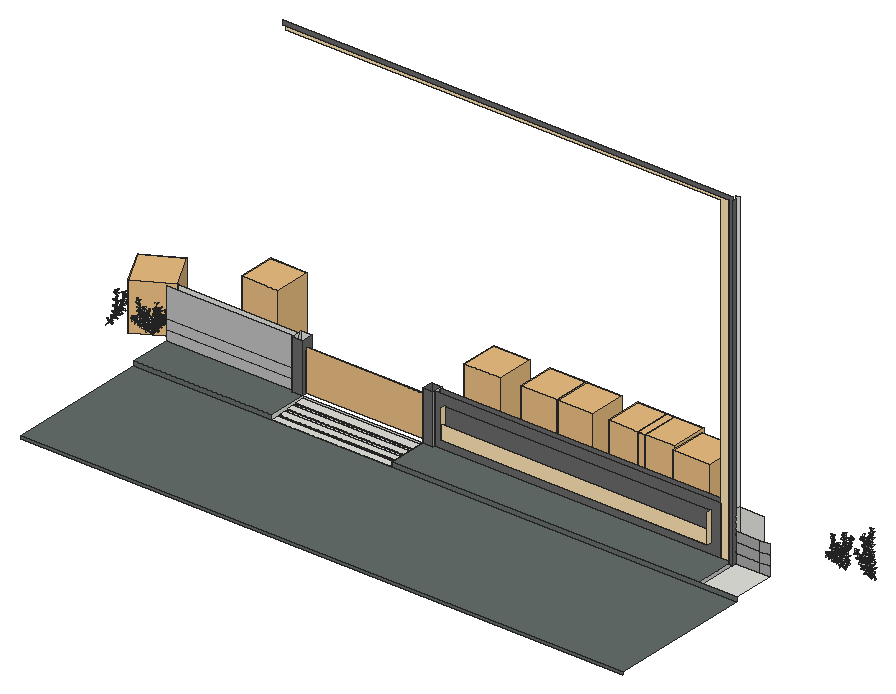
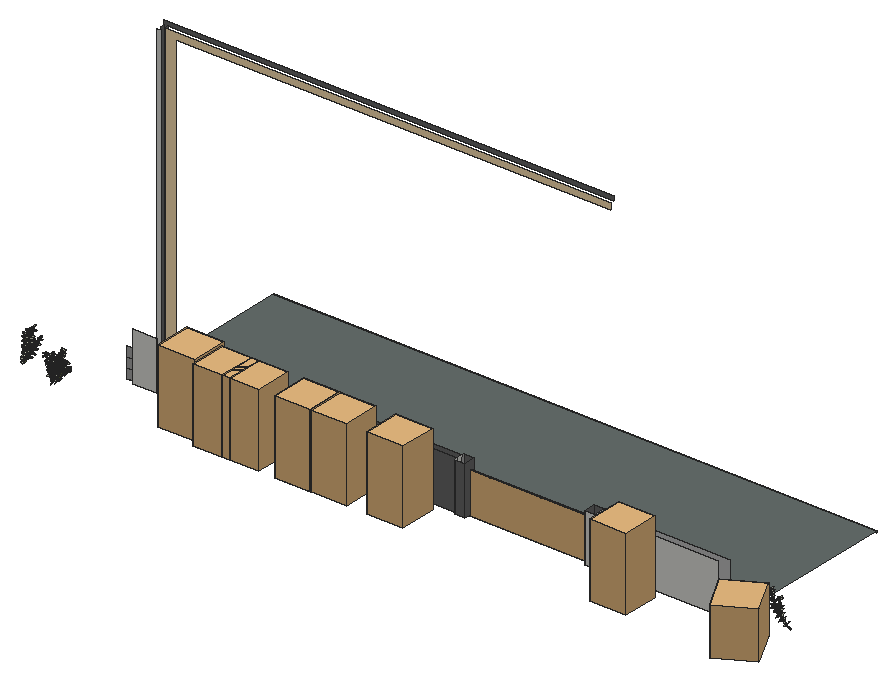
# SketchUp Ruby script. Lengths in inches.
U = 1.inch
M = Sketchup.active_model
def pt(a) = Geom::Point3d.new(a.map { |v| v * U })
def face(e, loops, mat)
  f = e.add_face(loops[0].map { |a| pt(a) })
  loops[1..].each { |l| e.add_face(l.map { |a| pt(a) }).erase! }
  f.material = f.back_material = mat if mat
  f
end
# faces: each face lists its corners as indices into pts; further lists are holes
def faces(e, pts, list, mat = nil) = list.each { |f| face(e, (f[0].is_a?(Array) ? f : [f]).map { |l| l.map { |i| pts[i] } }, mat) }
# xy, xz, yz: faces in a plane at the given z, y or x. An outline is a flat list of corners, or four numbers for a rectangle; further outlines are holes
def ring(l) = l.size == 4 ? [[l[0], l[1]], [l[2], l[1]], [l[2], l[3]], [l[0], l[3]]] : l.each_slice(2).to_a
def flat(e, list, mat, &to3) = list.each { |f| face(e, (f[0].is_a?(Array) ? f : [f]).map { |l| ring(l).map { |u, v| to3.(u, v) } }, mat) }
def xy(e, z, list, mat = nil) = flat(e, list, mat) { |x, y| [x, y, z] }
def xz(e, y, list, mat = nil) = flat(e, list, mat) { |x, z| [x, y, z] }
def yz(e, x, list, mat = nil) = flat(e, list, mat) { |y, z| [x, y, z] }
def lines(e, pts, list) = list.each { |a, b| e.add_line(pt(pts[a]), pt(pts[b])) }
# prism: a flat outline (further loops are holes) pulled along v
def prism(e, loops, v, mat = nil)
  f = face(e, loops, mat); d = Geom::Vector3d.new(v.map { |x| x * U })
  f.pushpull(f.normal.samedirection?(d) ? d.length : -d.length)
end
def box(e, o, s, mat = nil) = prism(e, [[o, [o[0] + s[0], o[1], o[2]], [o[0] + s[0], o[1] + s[1], o[2]], [o[0], o[1] + s[1], o[2]]]], [0, 0, s[2]], mat)
def at(x, y, z, deg = 0) = Geom::Transformation.translation(pt([x, y, z])) * Geom::Transformation.rotation(ORIGIN, Z_AXIS, deg.degrees)
def axes(o, x, y, z) = Geom::Transformation.new([*x, 0, *y, 0, *z, 0, *pt(o).to_a, 1])
def part(name) = M.definitions.add(name)
# library, detail: a bought-in or finely detailed component or shape, given as its bounding box
def library(name, o, s) = part(name).tap { |d| box(d.entities, o, s) }
def detail(e, o, s) = box(e.add_group.entities, o, s)
def put(e, d, t, mat = nil) = e.add_instance(d, t).tap { |i| i.material = mat if mat }
def group(e, t, mat = nil) = e.add_group.tap { |g| g.transformation = t; g.material = mat if mat }.entities
root = M.entities
M.materials.add("0ad16as01f6asdLeafVar1sfd015as60f1as6").color = [231, 235, 211]
M.materials.add("[0032_Moccasin]").color = [255, 228, 181]
M.materials.add("[0131_Silver]").color = [192, 192, 192]
M.materials.add("[0132_LightGray]").color = [169, 169, 169]
M.materials.add("[0134_DimGray]").color = [105, 105, 105]
M.materials.add("[Marble Carrara Gold Floor Tile]").color = [225, 223, 217]
M.materials.add("[Slate]").color = [102, 110, 108]
M.materials.add("asdfasdf0165f6asdLeafVar1sfd015as60f1as6").color = [231, 235, 211]
M.materials.add("dw_stemssadfasdfa0sdf1s01d6w1").color = [90, 97, 50]
c1 = part("vdw_leaf\#2")
p = [[0,0,0],[-2.77,1.61,2.32],[-4.3125,6.1,4.5],[-3.97,13.49,6.09],[-2.47,18.57,6.3],[-0.2,22.73,5.75],
  [2.54,19.66,6.85],[4.3,15.93,7.09],[5.03,7.6,5.43],[3.32,1.76,2.74]]
faces(c1.entities,p,[[0,1,2,3,4,5],[0,5,6,7,8,9]],"asdfasdf0165f6asdLeafVar1sfd015as60f1as6")
c2 = part("dg_branch_1\#2")
p = [[46.12,1.57,35.62],[46,5.42,35.41],[0.14,1.79,0.05],[0.26,-2.0625,0.27],[74.05,2.99,75.8],[74.11,5.28,75.58],
  [103.46,0.47,94.74],[104.03,2.92,94.84],[81.14,16.92,120.46],[81.2,18.78,120.24],[130.47,-5.6875,130.27],[130.58,-3.66,129.85],
  [80.82,34.4375,191.22],[80.64,35.93,190.9],[148.49,-14.56,203.24],[148.9,-12.8125,203.11],[81.08,37.95,226.93],[81.4,39.1,227.03],
  [157.45,-18.19,250.77],[157.7,-17.01,250.41]]
faces(c2.entities,p,[[0,1,2,3],[4,0,1],[4,1,5],[6,4,5],[6,5,7],[8,4,5],[8,5,9],[10,6,7],
  [10,7,11],[12,8,9],[12,9,13],[14,10,11],[14,11,15],[16,12,13],[16,13,17],[18,14,15],
  [18,15,19]],"dw_stemssadfasdfa0sdf1s01d6w1")
c3 = part("vdw_branch1\#3")
put(c3.entities,c1,axes([120.69,-2.42,117.31],[1.12221,-0.24063,-0.65809],[0.19207,1.24776,-0.12871],[0.65778,0.01392,1.11658]))
put(c3.entities,c1,axes([81,38.9,226.05],[0.7888,-0.58155,0],[0.48308,0.65523,0.47],[-0.28484,-0.38635,0.83138]))
put(c3.entities,c1,axes([78.08,12.69,106.05],[-1.43826,-0.02353,-0.03177],[0.0088,-1.31777,0.57755],[-0.03854,0.57714,1.31741]))
put(c3.entities,c1,axes([130.18,-4.73,130.41],[-0.38031,-1.29044,-0.11242],[1.20662,-0.31032,-0.51987],[0.47109,-0.24694,1.24081]))
put(c3.entities,c1,axes([157.08,-17.89,249.93],[-0.91355,0.40674,0],[-0.37496,-0.84216,0.38752],[0.15762,0.35401,0.92186]))
put(c3.entities,c1,axes([90.64,3.03,86.49],[0.32514,-0.85045,-0.99675],[0.69523,0.98247,-0.61148],[1.11061,-0.36604,0.67459]))
put(c3.entities,c1,axes([80.15,28.42,160.95],[-0.16039,0.95636,-1.06292],[-1.41646,0.03966,0.24943],[0.19509,1.07422,0.93709]))
put(c3.entities,c1,axes([126.74,-5.45,129.22],[-0.59819,0.96152,-0.6841],[-0.85772,0.12575,0.92675],[0.75427,0.88089,0.57856]))
put(c3.entities,c1,axes([133.22,-6.12,150.66],[-0.93823,0.76985,0.59124],[-0.47726,-1.08188,0.65135],[0.84525,0.24366,1.02405]))
put(c3.entities,c1,axes([80.43,22.89,141.32],[-1.42571,-0.19312,0.01373],[0.18338,-1.31425,0.5561],[-0.0621,0.5528,1.32692]))
put(c3.entities,c1,axes([33.14,0.88,26.42],[-0.13338,1.31536,0.04876],[-1.04528,-0.13221,0.7073],[0.72315,0.03348,1.07497]))
put(c3.entities,c1,axes([152.63,-15.08,221.76],[-1.28188,0.41945,0.0579],[-0.3638,-1.18547,0.53367],[0.21665,0.49113,1.23869]))
put(c3.entities,c1,axes([80.05,28.28,160.33],[-0.46732,-1.26661,0.40679],[1.27397,-0.40257,0.21004],[-0.07408,0.44645,1.30501]))
put(c3.entities,c1,axes([153.95,-14.8,235.875],[0.39005,1.07743,0.20605],[-0.96443,0.25296,0.50293],[0.42961,-0.3464,0.99807]))
put(c3.entities,c1,axes([80.2,24.22,141.74],[1.33062,-0.46576,0.02628],[0.44746,1.2746,-0.06608],[-0.00197,0.0722,1.37936]))
put(c3.entities,c1,axes([145.48,-12.5,188.92],[-1.32952,0.16983,0.16138],[-0.09299,-1.2361,0.53471],[0.21503,0.51548,1.22904]))
put(c3.entities,c1,axes([139.64,-9.18,171.24],[0.05682,1.30088,0.23414],[-1.13176,-0.05343,0.57151],[0.58357,-0.22963,1.13417]))
put(c3.entities,c1,axes([70.95,4.35,71.98],[-1.1081,-0.41873,0.64752],[0.33675,-1.28259,-0.25313],[0.6937,-0.04625,1.15721]))
put(c3.entities,c1,axes([59.85,4.55,56.17],[-0.26797,1.24526,0.35754],[-0.9369,-0.41634,0.74783],[0.83377,-0.10389,0.98674]))
put(c3.entities,c1,axes([33.11,3.36,25.66],[-0.57817,-1.07968,-0.5679],[1.11554,-0.21356,-0.7297],[0.49375,-0.78178,0.98363]))
put(c3.entities,c2,at(-0.21,0.34,-0.17),"dw_stemssadfasdfa0sdf1s01d6w1")
put(c3.entities,c1,axes([80.91,19.01,122.53],[-0.84258,1.13222,-0.27981],[-1.15093,-0.75138,0.42537],[0.18861,0.47293,1.3457]))
put(c3.entities,c1,axes([119.8,-1.22,114.1],[-1.3235,-0.25012,0.09101],[0.25933,-1.31572,0.15537],[0.05991,0.1698,1.33794]))
put(c3.entities,c1,axes([46.29,5.1,38.04],[0.98937,0.73827,-0.47585],[-0.72359,1.03721,0.10473],[0.44068,0.18581,1.20453]))
put(c3.entities,c1,axes([81.1875,33.03,184.45],[1.33883,0.26986,0.35053],[-0.09581,1.22087,-0.57399],[-0.42216,0.53228,1.20262]))
put(c3.entities,c1,axes([80.16,36.28,206.98],[-0.83993,0.85737,-0.6234],[-1.05964,-0.65701,0.5241],[0.02941,0.81391,1.07976]))
put(c3.entities,c1,axes([154.86,-16.15,234.87],[0.02509,-1.15302,-0.28506],[1.1487,-0.04894,0.29908],[-0.30202,-0.28195,1.11384]))
put(c3.entities,c1,axes([108.77,-0.33,101.14],[-0.47691,-1.03266,-0.72709],[1.25395,-0.29455,-0.40416],[0.15052,-0.81814,1.06325]))
put(c3.entities,c1,axes([89.79,3.01,85.87],[-0.61344,0.75518,0.8965],[-0.17758,-1.01824,0.73622],[1.13385,0.22574,0.58569]))
put(c3.entities,c1,axes([81.56,20.31,123.29],[0.37259,-1.3435,0.21057],[1.29385,0.32364,-0.22445],[0.16906,0.25791,1.34638]))
put(c3.entities,c1,axes([46.45,1.82,36.74],[-0.77883,0.29892,1.0614],[0.19124,-1.24314,0.49044],[1.08598,0.43329,0.67484]))
put(c3.entities,c1,axes([71.37,4.02,72.32],[0.72905,0.81546,-0.74421],[-0.66805,0.98958,0.42988],[0.8391,0.14186,0.97745]))
put(c3.entities,c1,axes([136.59,-5.88,150.53],[0.85845,-0.99897,-0.12437],[0.96526,0.81273,0.13453],[-0.02572,-0.18182,1.28292]))
put(c3.entities,c1,axes([80.375,38.8,225.86],[-0.25178,0.96778,0],[-0.89216,-0.23211,0.38752],[0.37503,0.09757,0.92186]))
put(c3.entities,c1,axes([74.43,7.99,85.38],[-1.05703,0.91669,-0.33543],[-0.95806,-0.87958,0.61531],[0.18697,0.6754,1.25659]))
put(c3.entities,c1,axes([76.57,9.74,89.32],[0.63146,-1.21538,0.33508],[1.18148,0.49387,-0.43517],[0.26321,0.48577,1.26593]))
put(c3.entities,c1,axes([81.6875,36.97,207.4],[0.09422,-1.04424,0.38486],[1.01646,0.1939,0.27727],[-0.33299,0.33382,0.98727]))
put(c3.entities,c1,axes([157.29,-17.17,249.98],[0.50586,-0.50586,0],[0.38853,0.38853,0.41105],[-0.29684,-0.29684,0.56115]))
put(c3.entities,c1,axes([79.92,15.8,106.09],[1.03917,-0.29343,-0.90675],[-0.14587,1.22131,-0.5624],[0.92163,0.5191,0.88824]))
put(c3.entities,c1,axes([61.95,3.88,56.26],[0.41243,-1.28546,0],[1.17466,0.37688,-0.54831],[0.5221,0.16751,1.23363]))
put(c3.entities,c1,axes([151.99,-14.79,208.15],[-0.48571,-1.21723,-0.32393],[1.25386,-0.50033,0],[-0.12005,-0.30087,1.31056]))
put(c3.entities,c1,axes([108.44,0.62,102.22],[0.82183,0.96078,0.38967],[-0.62327,0.08618,1.10203],[0.79141,-0.88661,0.51693]))
put(c3.entities,c1,axes([145.6,-10.56,188.62],[1.03241,-0.02554,-0.82693],[0.3944,1.11584,0.45794],[0.70325,-0.61672,0.89706]))
put(c3.entities,c1,axes([78.59,32.3,183.89],[-1.12675,-0.42036,0.43987],[0.5899,-0.98149,0.57312],[0.14901,0.70693,1.05726]))
put(c3.entities,c1,axes([152.08,-13.42,223.37],[0.79993,-0.44251,-0.69938],[0.68456,0.82615,0.26026],[0.41048,-0.60953,0.85515]))
put(c3.entities,c1,axes([140.71,-8.74,170.55],[0.41903,-1.24177,-0.32393],[1.26224,0.33728,0.33986],[-0.23168,-0.40836,1.26573]))
put(c3.entities,c1,axes([149.25,-12.53,205.78],[1.24456,0.38285,0.23414],[-0.42999,1.04826,0.57151],[-0.02056,-0.62679,1.13417]))
c4 = part("vdw_leaf\#3")
p = [[0,0,0],[-2.77,1.61,2.32],[-4.3125,6.1,4.5],[-3.97,13.49,6.09],[-2.47,18.57,6.3],[-0.2,22.73,5.75],
  [2.54,19.66,6.85],[4.3,15.93,7.09],[5.03,7.6,5.43],[3.32,1.76,2.74]]
faces(c4.entities,p,[[0,1,2,3,4,5],[0,5,6,7,8,9]],"asdfasdf0165f6asdLeafVar1sfd015as60f1as6")
c5 = part("dw_brancj_2\#2")
p = [[9.7,-0.22,29.95],[0.23,-1.96,0.34],[-0.05,1.51,0.11],[9.65,1.51,29.46],[18.64,-8.75,84.43],[18.96,-6.63,84.625],
  [1.53,6.02,63.68],[1.42,8.18,63.25],[-10.58,8.77,161.17],[-10.41,9.98,160.68],[26.34,-9.37,211.72],[26.57,-8.28,211.23]]
faces(c5.entities,p,[[0,1,2],[0,2,3],[4,0,3],[4,3,5],[6,0,3],[6,3,7],[8,6,7],[8,7,9],
  [10,4,5],[10,5,11]],"dw_stemssadfasdfa0sdf1s01d6w1")
c6 = part("vdw_branch2\#3")
put(c6.entities,c4,axes([19.53,-5.9,102.42],[1.12377,-0.50004,0],[0.46097,1.03596,0.47664],[-0.19377,-0.43548,1.13389]))
put(c6.entities,c4,axes([-5.89,6.52,109.44],[-1.07209,0.83679,0],[-0.77141,-0.98832,0.52702],[0.32427,0.41545,1.25373]))
put(c6.entities,c4,axes([-0.44,8.23,75.28],[0.88709,-0.9947,0],[0.92159,0.82189,0.33087],[-0.25219,-0.22491,1.26111]))
put(c6.entities,c4,axes([24.71,-8.97,190.81],[-0.82641,0.91101,0],[-0.83983,-0.76184,0.47664],[0.35303,0.32025,1.13389]))
put(c6.entities,c4,axes([-2.29,8.24,91.35],[1.24603,-0.47303,0],[0.43826,1.15445,0.33087],[-0.11993,-0.31592,1.26111]))
put(c6.entities,c4,axes([12.26,-3.11,37.92],[-0.64625,1.02205,0.22511],[-1.04383,-0.61044,-0.22511],[-0.07533,-0.30931,1.18809]))
put(c6.entities,c4,axes([26.17,-9.17,210.27],[-0.99452,-0.10453,0],[0.09636,-0.91681,0.38752],[-0.04051,0.38539,0.92186]))
put(c6.entities,c4,axes([-6.07,9.4,125.35],[-0.90214,-0.98107,0],[0.90896,-0.83583,0.33087],[-0.24874,0.22873,1.26111]))
put(c6.entities,c4,axes([-4.13,7.29,110.58],[0.44715,-1.078,0.64369],[1.05816,0.63649,0.33087],[-0.58725,0.40856,1.09216]))
put(c6.entities,c4,axes([23.91,-8.22,171.96],[0.62307,0.85009,-0.63406],[-0.71531,0.8798,0.47664],[0.78296,0.12729,0.94004]))
put(c6.entities,c5,at(-0.09,0.18,-0.25),"dw_stemssadfasdfa0sdf1s01d6w1")
put(c6.entities,c4,axes([23.34,-9.65,156.59],[-0.31364,-1.00782,0.58216],[1.10369,-0.17062,0.29925],[-0.17137,0.6239,0.98776]))
put(c6.entities,c4,axes([15.03,-3.37,58.83],[-1.05425,-0.00194,0.58442],[-0.14303,-1.11707,-0.26172],[0.55355,-0.3046,0.99755]))
put(c6.entities,c4,axes([-11.625,9.46,160.37],[0.36812,0.92978,0],[-0.85713,0.33936,0.38752],[0.3603,-0.14265,0.92186]))
put(c6.entities,c4,axes([21.32,-8.53,138.72],[1.21379,0.19904,0],[-0.19904,1.21379,0],[0,0,1.23]))
put(c6.entities,c4,axes([22.54,-9.2,141.43],[-1.02887,0.17955,0.60182],[-0.23387,-1.13057,-0.06253],[0.56696,-0.17376,1.02111]))
put(c6.entities,c4,axes([23.9,-8.82,173.84],[-1.14567,-0.37474,0],[0.35918,-1.0981,0.04438],[-0.01409,0.04308,1.17993]))
put(c6.entities,c4,axes([-7.84,8.92,143.59],[-1.26971,0.40522,0],[-0.37543,-1.17638,0.33087],[0.10274,0.32192,1.26111]))
put(c6.entities,c4,axes([19.77,-8.01,85.98],[-0.32405,-1.14591,0.18674],[1.10278,-0.32969,-0.10948],[0.15845,0.14442,1.16117]))
put(c6.entities,c4,axes([-0.62,5.76,76.34],[-0.08879,1.17576,-0.67771],[-1.34525,-0.16582,-0.11144],[-0.17897,0.66309,1.17383]))
put(c6.entities,c4,axes([20.49,-8.22,121.07],[0.39924,-0.78471,-0.8233],[1.08735,0.33121,0.2116],[0.09035,-0.83005,0.83495]))
put(c6.entities,c4,axes([15.15,-3.72,62.9],[1.16251,0.40128,-0.0211],[-0.39924,1.16074,0.07874],[0.0456,-0.06757,1.2273]))
put(c6.entities,c4,axes([20.72,-8.08,120.26],[-0.03693,1.2277,-0.06551],[-1.22944,-0.03698,0],[-0.00197,0.06548,1.22825]))
put(c6.entities,c4,axes([22.58,-8.36,155.57],[-0.56247,1.09386,0],[-1.00839,-0.51852,0.47664],[0.42389,0.21796,1.13389]))
put(c6.entities,c4,axes([3.97,3.13,57.96],[-1.09459,0.76041,0],[-0.72262,-1.0402,-0.1735],[-0.10109,-0.14552,1.29352]))
put(c6.entities,c4,axes([-10.8,9.06,160.75],[-0.66334,-0.72138,0],[0.66835,-0.61458,0.24329],[-0.1829,0.16818,0.92729]))
put(c6.entities,c4,axes([19.06,-9.3125,103.96],[-1.01345,0.25553,-0.60051],[-0.2265,-1.12952,-0.09839],[-0.59598,0.03076,1.01889]))
put(c6.entities,c4,axes([18.07,-6.2,81.7],[-0.56247,1.09386,0],[-1.00839,-0.51852,0.47664],[0.42389,0.21796,1.13389]))
put(c6.entities,c4,axes([12.95,-0.39,43.31],[0.13044,-1.19832,0],[1.11025,0.12085,0.29925],[-0.30382,-0.03307,1.14057]))
put(c6.entities,c4,axes([2.28,8.28,56.18],[1.32413,-0.31027,0],[0.30923,1.31968,-0.11144],[0.02542,0.1085,1.35543]))
put(c6.entities,c4,axes([-7.55,9.96,143.07],[1.34251,-0.21744,0],[0.20045,1.23761,0.52702],[-0.08426,-0.52024,1.25373]))
put(c6.entities,c4,axes([26.15,-8.25,210.66],[0.94661,-0.25364,0],[0.235,0.87703,0.24329],[-0.06431,-0.24,0.92729]))
put(c6.entities,c4,axes([-6.48,11.37,125.16],[0.64635,1.10315,0.46356],[-1.16569,0.46153,0.52702],[0.27017,-0.6478,1.16488]))
put(c6.entities,c4,axes([25.74,-8.35,191.28],[0.13044,-1.19832,0],[1.11025,0.12085,0.29925],[-0.30382,-0.03307,1.14057]))
put(c6.entities,c4,axes([-5.125,7.47,91.6],[-1.10024,0.63688,0.48318],[-0.78682,-1.00808,-0.46292],[0.14137,-0.65404,1.184]))
c7 = part("vdw_leaf\#1")
p = [[0,0,0],[-2.77,1.61,2.32],[-4.3125,6.1,4.5],[-3.97,13.49,6.09],[-2.47,18.57,6.3],[-0.2,22.73,5.75],
  [2.54,19.66,6.85],[4.3,15.93,7.09],[5.03,7.6,5.43],[3.32,1.76,2.74]]
faces(c7.entities,p,[[0,1,2,3,4,5],[0,5,6,7,8,9]],"0ad16as01f6asdLeafVar1sfd015as60f1as6")
c8 = part("dw_branch_3\#2")
p = [[-10.06,-1.6,62.9],[-0.2,1.54,-0.01],[-10.43,1.54,62.72],[0.18,-1.6,0.17],[-23.75,-21.66,88.91],[-25.7,-20.3,89.55],
  [13.4,11.62,104.56],[13.33,13.52,104.47],[-49.25,-41.87,130.3125],[-50.33,-40.21,130.71],[-4.97,21.13,143.98],[35.61,27.99,178.64],
  [-5.09,23.64,143.96],[35.32,29.14,178.46],[-67.7,-55.38,181.06],[-68.34,-54.45,181.62],[-22.8125,33.9,200.59],[-22.94,35.79,200.41],
  [56.61,36.78,229.75],[56.29,38.09,229.57],[-70.63,-67.46,248.85],[-70.72,-66.33,249.5],[-25.05,43.32,240.75],[-24.98,44.26,240.57]]
faces(c8.entities,p,[[0,1,2],[0,3,1],[4,2,5],[4,0,2],[6,0,2],[6,2,7],[8,4,5],[8,5,9],
  [10,6,7],[11,6,7],[10,7,12],[11,7,13],[14,8,9],[14,9,15],[16,10,12],[16,12,17],
  [18,11,13],[18,13,19],[20,14,15],[20,15,21],[22,16,17],[22,17,23]],"dw_stemssadfasdfa0sdf1s01d6w1")
c9 = part("dw_branch3\#2")
put(c9.entities,c7,axes([-70.33,-63.58,233.32],[-1.00752,0.412,0.78596],[-0.24851,-1.22189,0.32195],[0.83141,0.09817,1.01433]))
put(c9.entities,c7,axes([-66.93,-54.91,182.82],[-0.84976,-0.98359,0.33619],[0.99572,-0.74889,0.32577],[-0.05223,0.46521,1.22907]))
put(c9.entities,c7,axes([-46.12,-39.49,126.35],[1.23843,0.5364,0.23552],[-0.56438,0.94474,0.81599],[0.15707,-0.83465,1.07498]))
put(c9.entities,c7,axes([13.0625,13.13,104.77],[-1.01271,0.69982,-0.26884],[-0.74268,-0.99813,0.19939],[-0.10222,0.31872,1.21473]))
put(c9.entities,c7,axes([-18.87,30.42,186.42],[0.36309,1.06515,-0.56675],[-1.14134,0.49515,0.19939],[0.39128,0.45593,1.10754]))
put(c9.entities,c7,axes([-3.2,4.15,75.77],[-1.04153,0.55414,0.44243],[-0.23365,-1.01045,0.71554],[0.6695,0.50943,0.93801]))
put(c9.entities,c7,axes([23.2,19.41,136.3],[-0.65687,-1.11295,-0.05714],[1.05857,-0.61429,-0.20411],[0.15163,-0.1536,1.24868]))
put(c9.entities,c7,axes([-25.57,35.48,201.32],[-0.64726,0.62827,0.87973],[-0.71635,-1.0172,0.19939],[0.80962,-0.39773,0.87973]))
put(c9.entities,c7,axes([-36.37,-32.14,110.35],[-0.80747,1.09962,0.12544],[-0.83333,-0.50188,-0.96467],[-0.72833,-0.64487,0.96467]))
put(c9.entities,c7,axes([-9.89,26.72,156.79],[0.45529,1.02969,0.56572],[-1.16919,0.33753,0.32662],[0.11537,-0.64297,1.07744]))
put(c9.entities,c7,axes([-26.57,46.1,241.0625],[0.00015,0.80921,0.22536],[-0.83985,0.00446,-0.01542],[-0.01605,-0.22532,0.80906]))
put(c9.entities,c7,axes([-9.2,-2.58,61.06],[-1.10001,-0.40312,0.39014],[0.40883,-1.1116,0.00411],[0.35732,0.13566,1.14763]))
put(c9.entities,c7,axes([-69.91,-63.11,233.93],[1.36249,-0.1432,0],[0.13201,1.25603,0.5309],[-0.05549,-0.52799,1.26295]))
put(c9.entities,c7,axes([32.2,25.46,166.13],[0.06878,-1.29051,-0.05714],[1.22165,0.07415,-0.20411],[0.2113,-0.04403,1.24868]))
put(c9.entities,c7,axes([-5.68,-0.66,44.43],[-0.48448,-1.12287,0.17078],[0.98138,-0.33653,0.57135],[-0.48308,0.36756,1.04626]))
put(c9.entities,c7,axes([43.45,32.81,198.64],[0.5408,1.19584,0.14106],[-0.94242,0.32409,0.86557],[0.74952,-0.45533,0.98656]))
put(c9.entities,c7,axes([12.52,14.14,104.98],[1.02694,0.54888,0.41092],[-0.53566,1.05407,-0.06927],[-0.38969,-0.12321,1.13846]))
put(c9.entities,c7,axes([44.55,32.375,198.73],[-0.65687,-1.11295,-0.05714],[1.05857,-0.61429,-0.20411],[0.15163,-0.1536,1.24868]))
put(c9.entities,c7,axes([-5.67,21.17,141.44],[-1.10726,0.43603,-0.32953],[-0.49537,-1.03435,0.29588],[-0.17521,0.40597,1.12589]))
put(c9.entities,c7,axes([55.69,37.84,229.48],[0.18984,0.96334,0.18958],[-0.71996,0.0053,0.69399],[0.66755,-0.26823,0.69457]))
put(c9.entities,c7,axes([-21.52,36.85,205.2],[0.72606,-0.98817,0.14519],[0.94364,0.7084,0.10251],[-0.16885,0.05176,1.19664]))
put(c9.entities,c7,axes([-68.51,-56.35,196.07],[1.16319,0.72381,0],[-0.66725,1.0723,0.5309],[0.28049,-0.45075,1.26295]))
put(c9.entities,c8,at(0.01,-0.09,-0.02),"dw_stemssadfasdfa0sdf1s01d6w1")
put(c9.entities,c7,axes([-2.49,5.18,75.91],[0.78614,-0.90346,-0.30078],[0.86953,0.79562,-0.11715],[0.28546,-0.14014,1.16705]))
put(c9.entities,c7,axes([-23.125,-16.22,82.25],[0.32175,1.32576,0.12544],[-1.33153,0.31835,0.05068],[0.01989,-0.13382,1.3633]))
put(c9.entities,c7,axes([-23.75,41.99,230.3],[0.85958,-0.87451,0.14519],[0.66531,0.75721,0.62192],[-0.54076,-0.36226,1.01955]))
put(c9.entities,c7,axes([27.07,22.48,149.34],[0.92952,-0.64745,-0.62467],[0.50188,1.074,-0.36637],[0.71693,0.02135,1.04468]))
put(c9.entities,c7,axes([17.66,16.25,119.93],[-0.91649,0.83891,-0.3601],[-0.87434,-0.77966,0.40896],[0.0492,0.54447,1.14321]))
put(c9.entities,c7,axes([-68.37,-54.54,181.63],[0.32047,1.28399,0.35434],[-1.33153,0.31835,0.05068],[-0.03484,-0.35624,1.32241]))
put(c9.entities,c7,axes([-28.98,-27.1,96.48],[-0.8814,-0.35966,-0.98523],[0.75246,-1.11336,-0.26672],[-0.73065,-0.71272,0.91382]))
put(c9.entities,c7,axes([-15.23,28.43,172.72],[-1.21149,0.11898,0.32517],[-0.09739,-1.25259,0.09551],[0.33228,0.0667,1.21356]))
put(c9.entities,c7,axes([-17.5625,31.23,186.85],[-0.49275,-1.12287,0.14519],[0.95014,-0.33653,0.62192],[-0.53717,0.36756,1.01955]))
put(c9.entities,c7,axes([26.7,21.22,149.39],[-1.00104,0.22334,0.83093],[0.36894,-1.0402,0.72406],[0.77731,0.78134,0.72643]))
put(c9.entities,c7,axes([-31.125,-24.87,97.38],[0.75482,-0.86936,0.69068],[-0.00159,0.80023,1.00899],[-1.08766,-0.58016,0.45842]))
put(c9.entities,c7,axes([-71.21,-66.73,248.67],[0.25207,0.96771,0],[-0.8921,0.23237,0.38752],[0.375,-0.09768,0.92186]))
put(c9.entities,c7,axes([-24.11,41.05,229.55],[-1.11612,0.51924,-0.26884],[-0.56394,-1.10897,0.19939],[-0.15444,0.29694,1.21473]))
put(c9.entities,c7,axes([6.75,8.37,91.63],[-0.33418,-1.12287,0.39014],[1.13558,-0.33653,0.00411],[0.10478,0.36756,1.14763]))
put(c9.entities,c7,axes([-26,45.89,241.63],[-0.26986,-0.70824,-0.32129],[0.56818,-0.39091,0.38449],[-0.49365,-0.09775,0.63011]))
put(c9.entities,c7,axes([3.74,17.32,124.35],[0.22441,1.22913,-0.16274],[-1.07812,0.11178,-0.64246],[-0.61228,0.25367,1.07162]))
put(c9.entities,c7,axes([-5.44,22.27,140.88],[1.2203,0.00475,0.31374],[-0.097,1.20386,0.35905],[-0.29841,-0.37189,1.1663]))
put(c9.entities,c7,axes([-13.79,29.35,173.31],[0.83169,-0.90108,0.14519],[0.68877,0.73594,0.62192],[-0.55187,-0.34509,1.01955]))
put(c9.entities,c7,axes([-16.92,-7.26,72.98],[1.30647,0.30378,-0.27886],[0.07026,0.74892,1.14503],[0.40633,-1.10623,0.69861]))
put(c9.entities,c7,axes([4.8,17.55,125.22],[-0.25598,-1.17842,0.26559],[1.01553,-0.08455,0.60363],[-0.56975,0.35087,1.00767]))
put(c9.entities,c7,axes([5.3125,8.35,91.45],[0.00638,1.22913,-0.27714],[-1.16413,0.11178,0.46895],[0.48205,0.25367,1.13617]))
put(c9.entities,c7,axes([38.12,30.57,183.07],[1.12534,0.26182,-0.63833],[-0.46674,1.18829,-0.33545],[0.5081,0.51169,1.10563]))
put(c9.entities,c7,axes([-70.41,-60.38,214.47],[-0.41425,1.30587,0],[-1.20383,-0.38188,0.5309],[0.50605,0.16053,1.26295]))
put(c9.entities,c7,axes([37.03,28.75,180.67],[-1.12533,0.00102,-0.63799],[-0.00113,-1.2408,0],[-0.62497,0.00057,1.10237]))
put(c9.entities,c7,axes([30.71,25.35,165.96],[-0.1364,1.29314,0.22715],[-1.08768,-0.23921,0.70862],[0.73536,-0.11394,1.09026]))
put(c9.entities,c7,axes([-38.05,-30.84,110.67],[-0.31533,-1.27379,-0.2839],[1.018,-0.40311,0.67794],[-0.74394,-0.05723,1.08307]))
put(c9.entities,c7,axes([50.11,34.45,213.36],[-1.05669,0.74401,-0.05714],[-0.616,-0.82138,0.69675],[0.37221,0.60904,1.04705]))
put(c9.entities,c7,axes([-65.32,-58.78,200.07],[-1.14597,-0.19668,-0.6713],[0.21784,-1.26924,0],[-0.64812,-0.11124,1.139]))
put(c9.entities,c7,axes([-53.2,-43.37,143.59],[-0.72817,-1.09167,-0.2839],[0.82127,-0.72411,0.67794],[-0.71934,0.19815,1.08307]))
put(c9.entities,c7,axes([-61.1,-50.25,163.67],[-0.52887,1.19686,-0.30066],[-1.10762,-0.57104,-0.32484],[-0.42634,0.12264,1.23812]))
put(c9.entities,c7,axes([-54.12,-42.96,142.67],[0.32175,1.32576,0.12544],[-1.33153,0.31835,0.05068],[0.01989,-0.13382,1.3633]))
put(c9.entities,c7,axes([22.03,20.08,132.3],[1.17066,0.5058,-0.34078],[-0.35758,1.16671,0.50333],[0.49407,-0.35407,1.17172]))
put(c9.entities,c7,axes([-8.59,26.04,158.21],[-0.49275,-1.12287,0.14519],[0.95014,-0.33653,0.62192],[-0.53717,0.36756,1.01955]))
put(c9.entities,c7,axes([49.92,34.03,213.7],[1.24742,-0.35176,0.25024],[0.42127,1.159,-0.4708],[-0.09426,0.52477,1.20753]))
put(c9.entities,c7,axes([-70.34,-67.02,249.05],[-0.57048,-0.79684,0],[0.73827,-0.52855,0.24329],[-0.20203,0.14464,0.92729]))
put(c9.entities,c7,axes([56.04,36.81,228.63],[0.33451,-0.90845,-0.15237],[0.87636,0.33365,-0.06538],[0.11487,-0.11636,0.94597]))
put(c9.entities,c7,axes([-69.93,-60.58,214.88],[-0.45293,-0.99272,-0.78227],[1.14635,-0.58199,0.07483],[-0.40282,-0.65636,1.06615]))
put(c9.entities,c7,axes([-16.77,-8.59,72.7],[-1.22785,0.11509,0.53076],[-0.24879,-1.22495,-0.30991],[0.46742,-0.38989,1.16587]))
put(c9.entities,c7,axes([18.29,17.18,119.24],[1.19981,-0.45946,0.3029],[0.40159,1.22775,0.27158],[-0.37626,-0.1547,1.25575]))
put(c9.entities,c7,axes([-6.73,-0.68,43.74],[0.05346,1.22913,-0.27201],[-1.22696,0.11178,0.26396],[0.28163,0.25367,1.20164]))
put(c9.entities,c7,axes([-58.57,-48.42,160.98],[0.43385,-1.23789,0.39533],[1.04879,0.57965,0.66404],[-0.76727,0.09236,1.13122]))
put(c9.entities,c7,axes([-23.4,38.49,215.38],[0.06762,1.22913,-0.26884],[-1.23909,0.11178,0.19939],[0.21835,0.25367,1.21473]))
put(c9.entities,c7,axes([-22.21,-16.62,83.17],[-0.72817,-1.09167,-0.2839],[0.82127,-0.72411,0.67794],[-0.71934,0.19815,1.08307]))
put(c9.entities,c7,axes([-45.7,-40.77,126.53],[-1.33715,-0.0713,-0.0976],[0.07167,-1.28508,-0.04314],[-0.09306,-0.0492,1.31098]))
put(c9.entities,c7,axes([-22.39,38.51,216.12],[-0.49275,-1.12287,0.14519],[0.95014,-0.33653,0.62192],[-0.53717,0.36756,1.01955]))
c10 = library("Narrowleaf plant",[-0.44,-0.75,-1.28],[7.48,8.05,9.01])
c11 = library("plant",[-22.43,-22.29,0],[44.86,44.58,89.56])
c12 = library("DR 0003",[0,-1.57,0],[119.37,3.14,98.43])
c13 = library("Lamp Wall Outdoor 94-02",[-1.89,-4.65,-3.17],[3.78,4.65,6.35])
xy(root,-6,[[1338.625,0,2076.625,173.9375]],"[Slate]")
xy(root,-5.5,[[1507.11,173.9375,1654.31,182.83]])
xy(root,-5.4375,[[1507.11,182.83,1654.31,185.83]])
xy(root,-5.3125,[[1507.11,185.83,1654.31,194.72]],"[Marble Carrara Gold Floor Tile]")
xy(root,-4.8125,[[1507.11,194.72,1654.31,197.72]],"[Marble Carrara Gold Floor Tile]")
xy(root,-4.0625,[[1507.11,197.72,1654.31,206.61]],"[Marble Carrara Gold Floor Tile]")
xy(root,-3.5,[[1507.11,206.61,1654.31,209.61]],"[Marble Carrara Gold Floor Tile]")
xy(root,-2.75,[[1507.11,209.61,1654.31,221.5]],"[Marble Carrara Gold Floor Tile]")
xy(root,0,[[2036.3125,173.9375,2076.625,173.9375,2076.625,224.21,2065.6875,223.9375,2036.3125,223.9375],[2031.3125,218.9375,2036.3125,228.9375],[1494.42,221.5,1507.11,235.125],[1654.31,221.5,1666.62,235.125],[1443.61,223.9375,1494.42,231.9375],
  [1666.62,223.9375,2017.03,231.9375]])
xy(root,0,[[2031.3125,173.9375,2036.3125,218.9375]],"[0132_LightGray]")
xy(root,0,[[1338.625,173.9375,1507.11,173.9375,1507.11,221.5,1494.42,221.5,1494.42,223.9375,1338.625,223.9375],[1654.31,173.9375,2031.3125,173.9375,2031.3125,223.9375,1666.62,223.9375,1666.62,221.5,1654.31,221.5]],"[Slate]")
xy(root,12.32,[[1678.9375,218.9375,2004.71,223.9375]])
xz(root,0,[[1338.625,-9,2076.625,-6]],"[Slate]")
xz(root,173.9375,[[1338.625,-6,2076.625,-6,2076.625,0,1654.31,0,1654.31,-5.5,1507.11,-5.5,1507.11,0,1338.625,0]],"[Slate]")
xz(root,182.83,[[1507.11,-5.5,1654.31,-5.4375]])
xz(root,185.83,[[1507.11,-5.4375,1654.31,-5.3125]],"[Marble Carrara Gold Floor Tile]")
xz(root,194.72,[[1507.11,-5.3125,1654.31,-4.8125]],"[Marble Carrara Gold Floor Tile]")
xz(root,197.72,[[1507.11,-4.8125,1654.31,-4.0625]],"[Marble Carrara Gold Floor Tile]")
xz(root,206.61,[[1507.11,-4.0625,1654.31,-3.5]],"[Marble Carrara Gold Floor Tile]")
xz(root,209.61,[[1507.11,-3.5,1654.31,-2.75]],"[Marble Carrara Gold Floor Tile]")
xz(root,218.9375,[[1678.9375,12.32,2004.71,30]],"[0032_Moccasin]")
xz(root,218.9375,[[2031.3125,0,2036.3125,0,2036.3125,405.3125,1485.22,405.3125,1485.22,400.3125,2031.3125,400.3125]],"[0134_DimGray]")
xz(root,221.5,[[1494.42,0,1507.11,60],[1654.31,0,1666.62,60]],"[0134_DimGray]")
xz(root,221.5,[[1507.11,-2.75,1654.31,0]],"[Marble Carrara Gold Floor Tile]")
xz(root,223.9375,[[2017.03,0,2031.3125,0,2031.3125,400.3125,1485.22,400.3125,1485.22,392.3125,2017.03,392.3125]],"[0032_Moccasin]")
xz(root,223.9375,[[1338.625,0,1494.42,60]],"[0131_Silver]")
xz(root,223.9375,[[2036.3125,0,2065.6875,12],[2036.3125,12,2065.6875,24],[2036.3125,24,2065.6875,36]],"[0132_LightGray]")
xz(root,223.9375,[[[1666.62,0,2017.03,60],[1678.9375,12.32,2004.71,47.68]]],"[0134_DimGray]")
xz(root,228.9375,[[2031.3125,0,2036.3125,400.3125],[2036.3125,0,2065.5625,60]])
xz(root,231.9375,[[1346.625,0,1494.42,60]])
xz(root,231.9375,[[1666.62,0,2017.03,60]],"[0134_DimGray]")
xz(root,235.125,[[1494.42,0,1507.11,60]])
xz(root,235.125,[[1654.31,0,1666.62,60]],"[0134_DimGray]")
yz(root,1494.42,[[223.9375,0,231.9375,60],[231.9375,0,235.125,60]])
yz(root,1494.42,[[221.5,0,223.9375,60]],"[0134_DimGray]")
yz(root,1507.11,[[173.9375,-5.5,182.83,-5.5,182.83,-5.4375,185.83,-5.4375,185.83,-5.3125,194.72,-5.3125,194.72,-4.8125,197.72,-4.8125,197.72,-4.0625,206.61,-4.0625,206.61,-3.5,209.61,-3.5,209.61,-2.75,221.5,-2.75,221.5,0,173.9375,0]])
yz(root,1507.11,[[221.5,0,235.125,60]],"[0134_DimGray]")
yz(root,1654.31,[[173.9375,-5.5,173.9375,0,221.5,0,221.5,-2.75,209.61,-2.75,209.61,-3.5,206.61,-3.5,206.61,-4.0625,197.72,-4.0625,197.72,-4.8125,194.72,-4.8125,194.72,-5.3125,185.83,-5.3125,185.83,-5.4375,182.83,-5.4375,182.83,-5.5]])
yz(root,1654.31,[[221.5,0,235.125,60]],"[0134_DimGray]")
yz(root,1666.62,[[223.9375,0,231.9375,60],[231.9375,0,235.125,60]])
yz(root,1666.62,[[221.5,0,223.9375,60]],"[0132_LightGray]")
yz(root,1678.9375,[[218.9375,12.32,223.9375,47.68]],"[0032_Moccasin]")
yz(root,2004.71,[[218.9375,12.32,223.9375,47.68]],"[0032_Moccasin]")
yz(root,2017.03,[[223.9375,0,231.9375,60]])
yz(root,2031.3125,[[218.9375,0,223.9375,400.3125]],"[0134_DimGray]")
yz(root,2036.3125,[[223.9375,0,228.9375,60]])
yz(root,2036.3125,[[218.9375,0,223.9375,400.3125]],"[0134_DimGray]")
p = [[2076.625,224.21,0],[2076.625,224.21,12],[2065.6875,223.9375,12],[2065.6875,223.9375,0],[2065.6875,223.9375,24],[2076.625,224.21,24],
  [2065.6875,223.9375,36],[2076.625,224.21,36],[1491.42,223.9375,24],[1338.625,223.9375,24],[1491.42,223.9375,12],[1338.625,223.9375,12]]
faces(root,p,[[0,1,2,3],[4,2,1,5],[6,4,5,7]],"[0132_LightGray]")
lines(root,p,[[8,9],[10,11]])
put(root,c3,axes([1274.37,210.54,0.51],[0.11749,0.04939,0],[-0.04939,0.11749,0],[0,0,0.15683]))
put(root,c3,axes([1299.45,264.85,-3.7],[-0.07583,0.05409,0],[-0.05409,-0.07583,0],[0,0,0.11461]))
put(root,c6,axes([1297.39,263.99,-3.44],[-0.06851,-0.04024,-0.04853],[0.04493,-0.07649,0],[-0.03401,-0.01998,0.09777]))
put(root,c6,axes([1297.29,264.9,-2.94],[-0.10632,-0.02382,-0.02533],[0.02424,-0.1082,0],[-0.02009,-0.0045,0.13407]))
put(root,c9,axes([1301.4,267.54,-1.4],[0.06434,-0.05829,0.02833],[0.05722,0.06809,0.01535],[-0.02555,0.00573,0.10572]))
put(root,c9,axes([1302.21,263.1875,-5.91],[-0.0835,0.03705,-0.03198],[-0.01833,-0.07755,-0.06358],[-0.04138,-0.04041,0.09269]))
put(root,c9,axes([1300.44,262.77,-3.51],[0.11088,0,0],[0,0.11088,0],[0,0,0.13644]))
put(root,c10,axes([1292.62,228.46,1.02],[5.63682,3.11169,0],[-3.11169,5.63682,0],[0,0,6.43866]))
put(root,c3,axes([1309.74,235.01,-3.7],[-0.07583,0.05409,0],[-0.05409,-0.07583,0],[0,0,0.11461]))
put(root,c6,axes([1301.97,266.22,-4.3],[0.00659,0.0958,-0.06822],[-0.11062,0.0076,0],[0.0038,0.05531,0.11816]))
put(root,c3,axes([1300.13,262.92,-3.7],[0.01294,-0.09448,0],[0.09448,0.01294,0],[0,0,0.11734]))
put(root,c6,axes([1307.68,234.15,-3.44],[-0.06851,-0.04024,-0.04853],[0.04493,-0.07649,0],[-0.03401,-0.01998,0.09777]))
put(root,c6,axes([1307.59,235.07,-2.94],[-0.10632,-0.02382,-0.02533],[0.02424,-0.1082,0],[-0.02009,-0.0045,0.13407]))
put(root,c6,axes([1304.75,263.62,-4.8],[0.01852,0.08442,-0.0614],[-0.09748,0.02138,0],[0.01069,0.04874,0.10635]))
put(root,c9,axes([1311.6875,237.7,-1.4],[0.06434,-0.05829,0.02833],[0.05722,0.06809,0.01535],[-0.02555,0.00573,0.10572]))
put(root,c6,axes([1301.82,262.87,-4.91],[0.06689,-0.0646,-0.07431],[0.07703,0.07976,0],[0.04344,-0.04195,0.11443]))
put(root,c9,axes([1312.5,233.35,-5.91],[-0.0835,0.03705,-0.03198],[-0.01833,-0.07755,-0.06358],[-0.04138,-0.04041,0.09269]))
put(root,c6,axes([1305.37,263.17,-2.94],[0.10716,0.01972,-0.02533],[-0.02007,0.10905,0],[0.02025,0.00373,0.13407]))
put(root,c9,axes([1310.74,232.93,-3.51],[0.11088,0,0],[0,0.11088,0],[0,0,0.13644]))
put(root,c3,axes([1303.85,264.12,-3.7],[0.07973,0.03352,0],[-0.03352,0.07973,0],[0,0,0.10642]))
put(root,c6,axes([1312.26,236.38,-4.3],[0.00659,0.0958,-0.06822],[-0.11062,0.0076,0],[0.0038,0.05531,0.11816]))
put(root,c3,axes([1310.43,233.08,-3.7],[0.01294,-0.09448,0],[0.09448,0.01294,0],[0,0,0.11734]))
put(root,c6,axes([1315.05,233.79,-4.8],[0.01852,0.08442,-0.0614],[-0.09748,0.02138,0],[0.01069,0.04874,0.10635]))
put(root,c6,axes([1312.11,233.04,-4.91],[0.06689,-0.0646,-0.07431],[0.07703,0.07976,0],[0.04344,-0.04195,0.11443]))
put(root,c6,axes([1315.66,233.33,-2.94],[0.10716,0.01972,-0.02533],[-0.02007,0.10905,0],[0.02025,0.00373,0.13407]))
put(root,c3,axes([1314.15,234.29,-3.7],[0.07973,0.03352,0],[-0.03352,0.07973,0],[0,0,0.10642]))
put(root,c11,at(1437.87,264.68,0))
put(root,c12,axes([1507.11,227.75,0],[1.23315,0,0],[0,0.36,0],[0,0,0.5112]))
put(root,c11,at(1710.87,264.68,0))
put(root,c11,at(1780.31,264.68,0))
put(root,c11,at(1823.74,264.68,0))
put(root,c11,at(1887.68,264.68,0))
put(root,c13,at(1891.69,248.6,27.76))
put(root,c11,at(1923.31,264.68,0))
put(root,c11,at(1972.49,257.2,0))
put(root,c6,axes([2120.7,280.51,3.23],[-0.06851,-0.04024,-0.04853],[0.04493,-0.07649,0],[-0.03401,-0.01998,0.09777]))
put(root,c9,axes([2125.53,279.71,0.76],[-0.0835,0.03705,-0.03198],[-0.01833,-0.07755,-0.06358],[-0.04138,-0.04041,0.09269]))
put(root,c9,axes([2123.76,279.29,3.17],[0.11088,0,0],[0,0.11088,0],[0,0,0.13644]))
put(root,c3,axes([2123.45,279.45,2.97],[0.01294,-0.09448,0],[0.09448,0.01294,0],[0,0,0.11734]))
put(root,c6,axes([2125.14,279.4,1.76],[0.06689,-0.0646,-0.07431],[0.07703,0.07976,0],[0.04344,-0.04195,0.11443]))
put(root,c3,axes([2167.66,272.43,7.1875],[-0.11174,0.0797,0],[-0.0797,-0.11174,0],[0,0,0.16889]))
put(root,c6,axes([2164.62,271.16,7.57],[-0.10096,-0.0593,-0.07152],[0.0662,-0.11272,0],[-0.05012,-0.02944,0.14408]))
put(root,c6,axes([2164.48,272.51,8.3],[-0.15667,-0.0351,-0.03733],[0.03572,-0.15945,0],[-0.0296,-0.00663,0.19757]))
